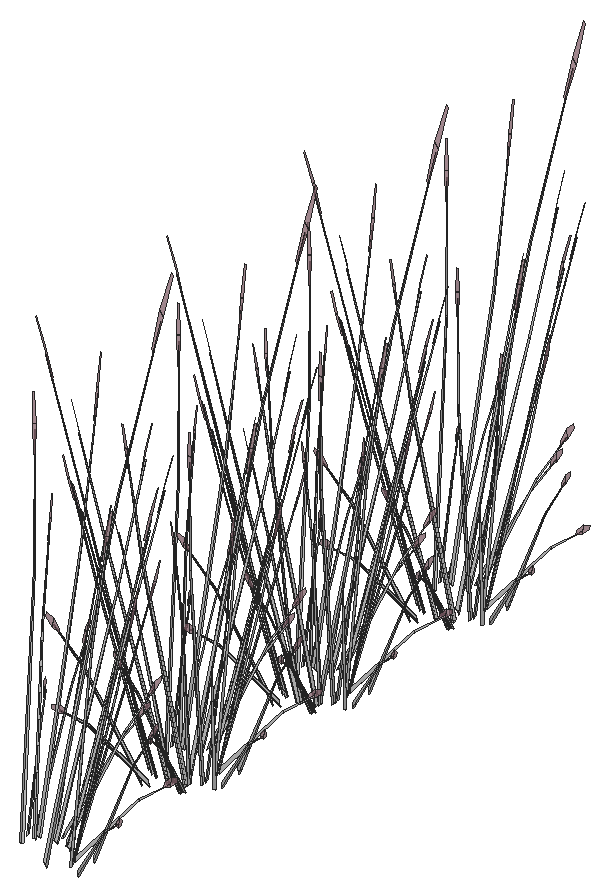
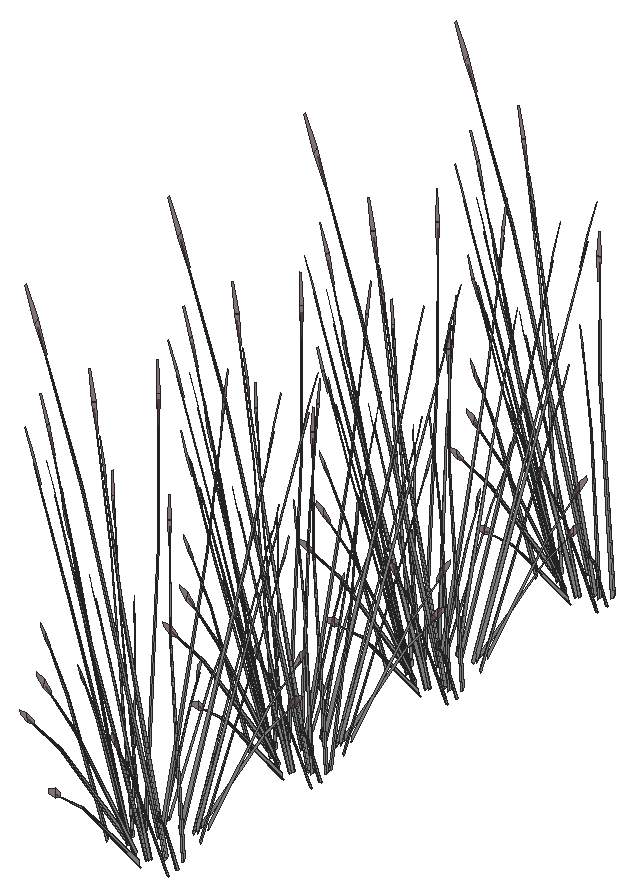
# SketchUp Ruby script. Lengths in inches.
U = 1.inch
M = Sketchup.active_model
def pt(a) = Geom::Point3d.new(a.map { |v| v * U })
def face(e, loops, mat)
  f = e.add_face(loops[0].map { |a| pt(a) })
  loops[1..].each { |l| e.add_face(l.map { |a| pt(a) }).erase! }
  f.material = f.back_material = mat if mat
  f
end
# faces: each face lists its corners as indices into pts; further lists are holes
def faces(e, pts, list, mat = nil) = list.each { |f| face(e, (f[0].is_a?(Array) ? f : [f]).map { |l| l.map { |i| pts[i] } }, mat) }
# xy, xz, yz: faces in a plane at the given z, y or x. An outline is a flat list of corners, or four numbers for a rectangle; further outlines are holes
def ring(l) = l.size == 4 ? [[l[0], l[1]], [l[2], l[1]], [l[2], l[3]], [l[0], l[3]]] : l.each_slice(2).to_a
def flat(e, list, mat, &to3) = list.each { |f| face(e, (f[0].is_a?(Array) ? f : [f]).map { |l| ring(l).map { |u, v| to3.(u, v) } }, mat) }
def xy(e, z, list, mat = nil) = flat(e, list, mat) { |x, y| [x, y, z] }
def xz(e, y, list, mat = nil) = flat(e, list, mat) { |x, z| [x, y, z] }
def yz(e, x, list, mat = nil) = flat(e, list, mat) { |y, z| [x, y, z] }
def lines(e, pts, list) = list.each { |a, b| e.add_line(pt(pts[a]), pt(pts[b])) }
# prism: a flat outline (further loops are holes) pulled along v
def prism(e, loops, v, mat = nil)
  f = face(e, loops, mat); d = Geom::Vector3d.new(v.map { |x| x * U })
  f.pushpull(f.normal.samedirection?(d) ? d.length : -d.length)
end
def box(e, o, s, mat = nil) = prism(e, [[o, [o[0] + s[0], o[1], o[2]], [o[0] + s[0], o[1] + s[1], o[2]], [o[0], o[1] + s[1], o[2]]]], [0, 0, s[2]], mat)
def at(x, y, z, deg = 0) = Geom::Transformation.translation(pt([x, y, z])) * Geom::Transformation.rotation(ORIGIN, Z_AXIS, deg.degrees)
def axes(o, x, y, z) = Geom::Transformation.new([*x, 0, *y, 0, *z, 0, *pt(o).to_a, 1])
def part(name) = M.definitions.add(name)
# library, detail: a bought-in or finely detailed component or shape, given as its bounding box
def library(name, o, s) = part(name).tap { |d| box(d.entities, o, s) }
def detail(e, o, s) = box(e.add_group.entities, o, s)
def put(e, d, t, mat = nil) = e.add_instance(d, t).tap { |i| i.material = mat if mat }
def group(e, t, mat = nil) = e.add_group.tap { |g| g.transformation = t; g.material = mat if mat }.entities
root = M.entities
M.materials.add("LightPink_Translucent").color = [144, 107, 117]
M.materials["LightPink_Translucent"].alpha = 0.75
M.materials.add("[_0053_Ivory_]").color = [200, 200, 200]
c1 = part("blade")
p = [[2.15,0.21,22],[0,0.17,0],[0.09,0.45,0],[2.18,0.31,22],[2.29,0.31,22],[0.38,0.45,0],
  [2.48,0.24,33],[2.49,0.24,33],[2.48,0.22,33]]
faces(c1.entities,p,[[0,1,2,3],[4,5,2,3],[6,3,4,7],[8,0,3,6]])
c2 = part("seeds")
p = [[0.3,-0.1,1.38],[-0.01,-0.03,1.59],[-0.01,-0.03,0.03],[0.14,-0.07,-0.07],[0.29,-0.03,3],[0.15,0.01,3.11]]
faces(c2.entities,p,[[0,1,2,3],[1,0,4,5]],"LightPink_Translucent")
c3 = part("blade with seeds")
put(c3.entities,c1,at(0,0,0))
put(c3.entities,c2,axes([2.4,0.25,30.99],[1.5799,-0.05474,1.17369],[-0.12525,1.92788,0.29478],[-0.07173,-0.02425,1.56792]))
put(root,c3,axes([648.13,153.46,131.37],[0.08428,-0.09579,1.74944],[-0.10787,-0.58756,-0.27667],[0.21147,-0.1114,0.14031]),"[_0053_Ivory_]")
put(root,c3,axes([646.47,154.35,131.6875],[-0.30559,-0.56943,-0.1216],[0.54237,-0.27983,-0.67495],[0.22856,-0.07513,1.02557]),"[_0053_Ivory_]")
put(root,c3,axes([646.72,154.34,131.38],[0.22307,0.42878,0.0643],[-0.40677,0.20987,0.50621],[0.17931,-0.04141,0.77189]),"[_0053_Ivory_]")
put(root,c3,axes([647.6875,156.04,131.36],[-0.05492,-0.05505,1.77383],[0.12013,-0.59013,-0.16761],[0.21632,-0.0377,0.31391]),"[_0053_Ivory_]")
put(root,c3,axes([645.79,155.53,131.6875],[0.03252,-0.63953,-0.1216],[0.61574,0.01748,-0.67495],[0.23714,0.04442,1.02557]),"[_0053_Ivory_]")
put(root,c3,axes([646.32,155.15,131.37],[0.13029,-0.01064,1.74944],[0.35737,-0.48855,-0.27667],[0.23175,0.06449,0.14031]),"[_0053_Ivory_]")
put(root,c3,axes([646.01,155.64,131.38],[-0.03058,0.47819,0.0643],[-0.4618,-0.01311,0.50621],[0.1769,0.05004,0.77189]),"[_0053_Ivory_]")
put(root,c3,axes([644.98,153.05,131.13],[-0.52482,-0.32674,1.38283],[0.55416,-0.50872,0.59665],[0.16933,0.30658,1.33663]),"[_0053_Ivory_]")
put(root,c3,axes([641.2,154.43,131.6875],[0.56181,0.34675,-0.1216],[-0.32367,0.50216,-0.67495],[-0.15873,0.17455,1.02557]),"[_0053_Ivory_]")
put(root,c3,axes([644.57,156.23,131.6875],[0.36191,-0.53827,-0.1216],[0.52412,0.3101,-0.67495],[0.18219,0.15207,1.02557]),"[_0053_Ivory_]")
put(root,c3,axes([644.1,156.68,131.36],[0.0018,-0.07613,1.77383],[0.52048,-0.3359,-0.16761],[0.18079,0.11989,0.31391]),"[_0053_Ivory_]")
put(root,c3,axes([641.82,155.8,131.38],[-0.49911,-0.0293,0.0643],[0.01368,-0.44245,0.50621],[-0.05223,0.16948,0.77189]),"[_0053_Ivory_]")
put(root,c3,axes([644.71,156.43,131.38],[-0.27604,0.39948,0.0643],[-0.39309,-0.23258,0.50621],[0.12709,0.12808,0.77189]),"[_0053_Ivory_]")
put(root,c3,axes([643.18,156.49,131.38],[-0.44753,0.21372,0.0643],[-0.21905,-0.38973,0.50621],[0.04322,0.1718,0.77189]),"[_0053_Ivory_]")
put(root,c3,axes([640.56,155.875,131.37],[-0.0151,0.12444,1.74944],[0.42844,0.43292,-0.27667],[-0.11216,0.20472,0.14031]),"[_0053_Ivory_]")
put(root,c3,axes([641.93,155.59,132.05],[0.6675,0.03116,-0.13498],[-0.01824,0.58993,-0.74919],[-0.04637,0.2272,1.13838]),"[_0053_Ivory_]")
put(root,c3,axes([643.16,156.25,131.6875],[0.59433,-0.29278,-0.1216],[0.29207,0.51964,-0.67495],[0.07842,0.21898,1.02557]),"[_0053_Ivory_]")
put(root,c3,axes([640.51,157.15,131.36],[0.0689,-0.03797,1.77383],[0.5695,0.25254,-0.16761],[-0.01338,0.21027,0.31391]),"[_0053_Ivory_]")
put(root,c3,axes([643.02,157.41,131.37],[0.07699,0.10127,1.74944],[0.6213,0.03978,-0.27667],[0.06248,0.22333,0.14031]),"[_0053_Ivory_]")
put(root,c3,axes([643.55,168.3,131.37],[-0.0929,-0.08817,1.74944],[-0.61994,0.0559,-0.27667],[-0.09894,-0.21089,0.14031]),"[_0053_Ivory_]")
put(root,c3,axes([646.33,169.38,131.37],[-0.00586,-0.12516,1.74944],[-0.49517,-0.36172,-0.27667],[0.07656,-0.21927,0.14031]),"[_0053_Ivory_]")
put(root,c3,axes([646.2,168.93,131.36],[-0.06168,0.04803,1.77383],[-0.60432,-0.16205,-0.16761],[-0.02188,-0.20961,0.31391]),"[_0053_Ivory_]")
put(root,c3,axes([642.91,168.01,131.36],[-0.01133,0.07538,1.77383],[-0.55883,0.27355,-0.16761],[-0.16445,-0.13983,0.31391]),"[_0053_Ivory_]")
put(root,c3,axes([644.49,169.66,131.6875],[-0.59433,0.29278,-0.1216],[-0.29207,-0.51964,-0.67495],[-0.07842,-0.21898,1.02557]),"[_0053_Ivory_]")
put(root,c3,axes([645.72,170.32,131.6875],[-0.6675,-0.03116,-0.1216],[0.01824,-0.58993,-0.67495],[0.04637,-0.2272,1.02557]),"[_0053_Ivory_]")
put(root,c3,axes([644.48,169.43,131.38],[0.44753,-0.21372,0.0643],[0.21905,0.38973,0.50621],[-0.04322,-0.1718,0.77189]),"[_0053_Ivory_]")
put(root,c3,axes([642.94,169.49,131.38],[0.27604,-0.39948,0.0643],[0.39309,0.23258,0.50621],[-0.12709,-0.12808,0.77189]),"[_0053_Ivory_]")
put(root,c3,axes([643.07,169.44,132.08],[-0.40534,0.60286,-0.13619],[-0.58702,-0.34732,-0.75594],[-0.20405,-0.17032,1.14864]),"[_0053_Ivory_]")
put(root,c3,axes([645.84,170.11,131.38],[0.49911,0.0293,0.0643],[-0.01368,0.44245,0.50621],[0.05223,-0.16948,0.77189]),"[_0053_Ivory_]")
put(root,c3,axes([646.45,171.48,131.6875],[-0.56181,-0.34675,-0.1216],[0.32367,-0.50216,-0.67495],[0.15873,-0.17455,1.02557]),"[_0053_Ivory_]")
put(root,c3,axes([647.83,171.33,131.36],[-0.07933,-0.00478,1.77383],[-0.32942,-0.51175,-0.16761],[0.13229,-0.16826,0.31391]),"[_0053_Ivory_]")
put(root,c3,axes([641.65,170.27,131.38],[0.03058,-0.47819,0.0643],[0.4618,0.01311,0.50621],[-0.1769,-0.05004,0.77189]),"[_0053_Ivory_]")
put(root,c3,axes([646.66,171.35,131.38],[0.41695,0.26447,0.0643],[-0.24275,0.37662,0.50621],[0.13368,-0.12176,0.77189]),"[_0053_Ivory_]")
put(root,c3,axes([648.13,171.94,131.37],[0.08428,-0.09579,1.74944],[-0.10787,-0.58756,-0.27667],[0.21147,-0.1114,0.14031]),"[_0053_Ivory_]")
put(root,c3,axes([646.47,172.83,131.6875],[-0.30559,-0.56943,-0.1216],[0.54237,-0.27983,-0.67495],[0.22856,-0.07513,1.02557]),"[_0053_Ivory_]")
put(root,c3,axes([646.72,172.82,131.38],[0.22307,0.42878,0.0643],[-0.40677,0.20987,0.50621],[0.17931,-0.04141,0.77189]),"[_0053_Ivory_]")
put(root,c3,axes([647.6875,174.53,131.36],[-0.05492,-0.05505,1.77383],[0.12013,-0.59013,-0.16761],[0.21632,-0.0377,0.31391]),"[_0053_Ivory_]")
put(root,c3,axes([645.79,174.02,131.6875],[0.03252,-0.63953,-0.1216],[0.61574,0.01748,-0.67495],[0.23714,0.04442,1.02557]),"[_0053_Ivory_]")
put(root,c3,axes([646.32,173.63,131.37],[0.13029,-0.01064,1.74944],[0.35737,-0.48855,-0.27667],[0.23175,0.06449,0.14031]),"[_0053_Ivory_]")
put(root,c3,axes([646.01,174.12,131.38],[-0.03058,0.47819,0.0643],[-0.4618,-0.01311,0.50621],[0.1769,0.05004,0.77189]),"[_0053_Ivory_]")
put(root,c3,axes([644.98,171.54,131.13],[-0.52482,-0.32674,1.38283],[0.55416,-0.50872,0.59665],[0.16933,0.30658,1.33663]),"[_0053_Ivory_]")
put(root,c3,axes([641.2,172.92,131.6875],[0.56181,0.34675,-0.1216],[-0.32367,0.50216,-0.67495],[-0.15873,0.17455,1.02557]),"[_0053_Ivory_]")
put(root,c3,axes([644.57,174.71,131.6875],[0.36191,-0.53827,-0.1216],[0.52412,0.3101,-0.67495],[0.18219,0.15207,1.02557]),"[_0053_Ivory_]")
put(root,c3,axes([644.1,175.16,131.36],[0.0018,-0.07613,1.77383],[0.52048,-0.3359,-0.16761],[0.18079,0.11989,0.31391]),"[_0053_Ivory_]")
put(root,c3,axes([641.82,174.29,131.38],[-0.49911,-0.0293,0.0643],[0.01368,-0.44245,0.50621],[-0.05223,0.16948,0.77189]),"[_0053_Ivory_]")
put(root,c3,axes([644.71,174.91,131.38],[-0.27604,0.39948,0.0643],[-0.39309,-0.23258,0.50621],[0.12709,0.12808,0.77189]),"[_0053_Ivory_]")
put(root,c3,axes([643.18,174.97,131.38],[-0.44753,0.21372,0.0643],[-0.21905,-0.38973,0.50621],[0.04322,0.1718,0.77189]),"[_0053_Ivory_]")
put(root,c3,axes([640.56,174.36,131.37],[-0.0151,0.12444,1.74944],[0.42844,0.43292,-0.27667],[-0.11216,0.20472,0.14031]),"[_0053_Ivory_]")
put(root,c3,axes([641.93,174.08,132.05],[0.6675,0.03116,-0.13498],[-0.01824,0.58993,-0.74919],[-0.04637,0.2272,1.13838]),"[_0053_Ivory_]")
put(root,c3,axes([643.16,174.73,131.6875],[0.59433,-0.29278,-0.1216],[0.29207,0.51964,-0.67495],[0.07842,0.21898,1.02557]),"[_0053_Ivory_]")
put(root,c3,axes([640.51,175.63,131.36],[0.0689,-0.03797,1.77383],[0.5695,0.25254,-0.16761],[-0.01338,0.21027,0.31391]),"[_0053_Ivory_]")
put(root,c3,axes([643.02,175.9,131.37],[0.07699,0.10127,1.74944],[0.6213,0.03978,-0.27667],[0.06248,0.22333,0.14031]),"[_0053_Ivory_]")
put(root,c3,axes([643.55,185.06,131.37],[-0.0929,-0.08817,1.74944],[-0.61994,0.0559,-0.27667],[-0.09894,-0.21089,0.14031]),"[_0053_Ivory_]")
put(root,c3,axes([646.33,186.14,131.37],[-0.00586,-0.12516,1.74944],[-0.49517,-0.36172,-0.27667],[0.07656,-0.21927,0.14031]),"[_0053_Ivory_]")
put(root,c3,axes([646.2,185.69,131.36],[-0.06168,0.04803,1.77383],[-0.60432,-0.16205,-0.16761],[-0.02188,-0.20961,0.31391]),"[_0053_Ivory_]")
put(root,c3,axes([642.91,184.77,131.36],[-0.01133,0.07538,1.77383],[-0.55883,0.27355,-0.16761],[-0.16445,-0.13983,0.31391]),"[_0053_Ivory_]")
put(root,c3,axes([644.49,186.42,131.6875],[-0.59433,0.29278,-0.1216],[-0.29207,-0.51964,-0.67495],[-0.07842,-0.21898,1.02557]),"[_0053_Ivory_]")
put(root,c3,axes([645.72,187.08,131.6875],[-0.6675,-0.03116,-0.1216],[0.01824,-0.58993,-0.67495],[0.04637,-0.2272,1.02557]),"[_0053_Ivory_]")
put(root,c3,axes([644.48,186.1875,131.38],[0.44753,-0.21372,0.0643],[0.21905,0.38973,0.50621],[-0.04322,-0.1718,0.77189]),"[_0053_Ivory_]")
put(root,c3,axes([642.94,186.25,131.38],[0.27604,-0.39948,0.0643],[0.39309,0.23258,0.50621],[-0.12709,-0.12808,0.77189]),"[_0053_Ivory_]")
put(root,c3,axes([643.07,186.2,132.08],[-0.40534,0.60286,-0.13619],[-0.58702,-0.34732,-0.75594],[-0.20405,-0.17032,1.14864]),"[_0053_Ivory_]")
put(root,c3,axes([645.84,186.87,131.38],[0.49911,0.0293,0.0643],[-0.01368,0.44245,0.50621],[0.05223,-0.16948,0.77189]),"[_0053_Ivory_]")
put(root,c3,axes([646.45,188.24,131.6875],[-0.56181,-0.34675,-0.1216],[0.32367,-0.50216,-0.67495],[0.15873,-0.17455,1.02557]),"[_0053_Ivory_]")
put(root,c3,axes([647.83,188.09,131.36],[-0.07933,-0.00478,1.77383],[-0.32942,-0.51175,-0.16761],[0.13229,-0.16826,0.31391]),"[_0053_Ivory_]")
put(root,c3,axes([641.65,187.03,131.38],[0.03058,-0.47819,0.0643],[0.4618,0.01311,0.50621],[-0.1769,-0.05004,0.77189]),"[_0053_Ivory_]")
put(root,c3,axes([646.66,188.11,131.38],[0.41695,0.26447,0.0643],[-0.24275,0.37662,0.50621],[0.13368,-0.12176,0.77189]),"[_0053_Ivory_]")
put(root,c3,axes([648.13,188.7,131.37],[0.08428,-0.09579,1.74944],[-0.10787,-0.58756,-0.27667],[0.21147,-0.1114,0.14031]),"[_0053_Ivory_]")
put(root,c3,axes([646.47,189.59,131.6875],[-0.30559,-0.56943,-0.1216],[0.54237,-0.27983,-0.67495],[0.22856,-0.07513,1.02557]),"[_0053_Ivory_]")
put(root,c3,axes([646.72,189.58,131.38],[0.22307,0.42878,0.0643],[-0.40677,0.20987,0.50621],[0.17931,-0.04141,0.77189]),"[_0053_Ivory_]")
put(root,c3,axes([647.6875,191.28,131.36],[-0.05492,-0.05505,1.77383],[0.12013,-0.59013,-0.16761],[0.21632,-0.0377,0.31391]),"[_0053_Ivory_]")
put(root,c3,axes([645.79,190.78,131.6875],[0.03252,-0.63953,-0.1216],[0.61574,0.01748,-0.67495],[0.23714,0.04442,1.02557]),"[_0053_Ivory_]")
put(root,c3,axes([646.32,190.39,131.37],[0.13029,-0.01064,1.74944],[0.35737,-0.48855,-0.27667],[0.23175,0.06449,0.14031]),"[_0053_Ivory_]")
put(root,c3,axes([641,189.8,131.38],[-0.41695,-0.26447,0.0643],[0.24275,-0.37662,0.50621],[-0.13368,0.12176,0.77189]),"[_0053_Ivory_]")
put(root,c3,axes([646.01,190.88,131.38],[-0.03058,0.47819,0.0643],[-0.4618,-0.01311,0.50621],[0.1769,0.05004,0.77189]),"[_0053_Ivory_]")
put(root,c3,axes([644.98,188.3,131.13],[-0.52482,-0.32674,1.38283],[0.55416,-0.50872,0.59665],[0.16933,0.30658,1.33663]),"[_0053_Ivory_]")
put(root,c3,axes([641.2,189.67,131.6875],[0.56181,0.34675,-0.1216],[-0.32367,0.50216,-0.67495],[-0.15873,0.17455,1.02557]),"[_0053_Ivory_]")
put(root,c3,axes([644.57,191.47,131.6875],[0.36191,-0.53827,-0.1216],[0.52412,0.3101,-0.67495],[0.18219,0.15207,1.02557]),"[_0053_Ivory_]")
put(root,c3,axes([644.1,191.92,131.36],[0.0018,-0.07613,1.77383],[0.52048,-0.3359,-0.16761],[0.18079,0.11989,0.31391]),"[_0053_Ivory_]")
put(root,c3,axes([641.82,191.05,131.38],[-0.49911,-0.0293,0.0643],[0.01368,-0.44245,0.50621],[-0.05223,0.16948,0.77189]),"[_0053_Ivory_]")
put(root,c3,axes([644.71,191.67,131.38],[-0.27604,0.39948,0.0643],[-0.39309,-0.23258,0.50621],[0.12709,0.12808,0.77189]),"[_0053_Ivory_]")
put(root,c3,axes([643.18,191.73,131.38],[-0.44753,0.21372,0.0643],[-0.21905,-0.38973,0.50621],[0.04322,0.1718,0.77189]),"[_0053_Ivory_]")
put(root,c3,axes([640.56,191.12,131.37],[-0.0151,0.12444,1.74944],[0.42844,0.43292,-0.27667],[-0.11216,0.20472,0.14031]),"[_0053_Ivory_]")
put(root,c3,axes([641.93,190.84,132.05],[0.6675,0.03116,-0.13498],[-0.01824,0.58993,-0.74919],[-0.04637,0.2272,1.13838]),"[_0053_Ivory_]")
put(root,c3,axes([643.16,191.49,131.6875],[0.59433,-0.29278,-0.1216],[0.29207,0.51964,-0.67495],[0.07842,0.21898,1.02557]),"[_0053_Ivory_]")
put(root,c3,axes([640.51,192.39,131.36],[0.0689,-0.03797,1.77383],[0.5695,0.25254,-0.16761],[-0.01338,0.21027,0.31391]),"[_0053_Ivory_]")
put(root,c3,axes([643.02,192.66,131.37],[0.07699,0.10127,1.74944],[0.6213,0.03978,-0.27667],[0.06248,0.22333,0.14031]),"[_0053_Ivory_]")
put(root,c3,axes([643.55,202.65,131.37],[-0.0929,-0.08817,1.74944],[-0.61994,0.0559,-0.27667],[-0.09894,-0.21089,0.14031]),"[_0053_Ivory_]")
put(root,c3,axes([646.33,203.73,131.37],[-0.00586,-0.12516,1.74944],[-0.49517,-0.36172,-0.27667],[0.07656,-0.21927,0.14031]),"[_0053_Ivory_]")
put(root,c3,axes([646.2,203.28,131.36],[-0.06168,0.04803,1.77383],[-0.60432,-0.16205,-0.16761],[-0.02188,-0.20961,0.31391]),"[_0053_Ivory_]")
put(root,c3,axes([642.91,202.36,131.36],[-0.01133,0.07538,1.77383],[-0.55883,0.27355,-0.16761],[-0.16445,-0.13983,0.31391]),"[_0053_Ivory_]")
put(root,c3,axes([644.49,204.01,131.6875],[-0.59433,0.29278,-0.1216],[-0.29207,-0.51964,-0.67495],[-0.07842,-0.21898,1.02557]),"[_0053_Ivory_]")
put(root,c3,axes([645.72,204.67,131.6875],[-0.6675,-0.03116,-0.1216],[0.01824,-0.58993,-0.67495],[0.04637,-0.2272,1.02557]),"[_0053_Ivory_]")
put(root,c3,axes([642.94,203.84,131.38],[0.27604,-0.39948,0.0643],[0.39309,0.23258,0.50621],[-0.12709,-0.12808,0.77189]),"[_0053_Ivory_]")
put(root,c3,axes([643.07,203.8,132.08],[-0.40534,0.60286,-0.13619],[-0.58702,-0.34732,-0.75594],[-0.20405,-0.17032,1.14864]),"[_0053_Ivory_]")
put(root,c3,axes([646.45,205.83,131.6875],[-0.56181,-0.34675,-0.1216],[0.32367,-0.50216,-0.67495],[0.15873,-0.17455,1.02557]),"[_0053_Ivory_]")
put(root,c3,axes([647.83,205.68,131.36],[-0.07933,-0.00478,1.77383],[-0.32942,-0.51175,-0.16761],[0.13229,-0.16826,0.31391]),"[_0053_Ivory_]")
put(root,c3,axes([641.65,204.625,131.38],[0.03058,-0.47819,0.0643],[0.4618,0.01311,0.50621],[-0.1769,-0.05004,0.77189]),"[_0053_Ivory_]")
put(root,c3,axes([646.66,205.7,131.38],[0.41695,0.26447,0.0643],[-0.24275,0.37662,0.50621],[0.13368,-0.12176,0.77189]),"[_0053_Ivory_]")
put(root,c3,axes([648.13,206.29,131.37],[0.08428,-0.09579,1.74944],[-0.10787,-0.58756,-0.27667],[0.21147,-0.1114,0.14031]),"[_0053_Ivory_]")
put(root,c3,axes([646.47,207.18,131.6875],[-0.30559,-0.56943,-0.1216],[0.54237,-0.27983,-0.67495],[0.22856,-0.07513,1.02557]),"[_0053_Ivory_]")
put(root,c3,axes([646.72,207.17,131.38],[0.22307,0.42878,0.0643],[-0.40677,0.20987,0.50621],[0.17931,-0.04141,0.77189]),"[_0053_Ivory_]")
put(root,c3,axes([647.6875,208.875,131.36],[-0.05492,-0.05505,1.77383],[0.12013,-0.59013,-0.16761],[0.21632,-0.0377,0.31391]),"[_0053_Ivory_]")
put(root,c3,axes([645.79,208.37,131.6875],[0.03252,-0.63953,-0.1216],[0.61574,0.01748,-0.67495],[0.23714,0.04442,1.02557]),"[_0053_Ivory_]")
put(root,c3,axes([646.32,207.98,131.37],[0.13029,-0.01064,1.74944],[0.35737,-0.48855,-0.27667],[0.23175,0.06449,0.14031]),"[_0053_Ivory_]")
put(root,c3,axes([644.98,205.89,131.13],[-0.52482,-0.32674,1.38283],[0.55416,-0.50872,0.59665],[0.16933,0.30658,1.33663]),"[_0053_Ivory_]")
put(root,c3,axes([641.2,207.27,131.6875],[0.56181,0.34675,-0.1216],[-0.32367,0.50216,-0.67495],[-0.15873,0.17455,1.02557]),"[_0053_Ivory_]")
put(root,c3,axes([644.57,209.0625,131.6875],[0.36191,-0.53827,-0.1216],[0.52412,0.3101,-0.67495],[0.18219,0.15207,1.02557]),"[_0053_Ivory_]")
put(root,c3,axes([644.1,209.51,131.36],[0.0018,-0.07613,1.77383],[0.52048,-0.3359,-0.16761],[0.18079,0.11989,0.31391]),"[_0053_Ivory_]")
put(root,c3,axes([643.18,209.32,131.38],[-0.44753,0.21372,0.0643],[-0.21905,-0.38973,0.50621],[0.04322,0.1718,0.77189]),"[_0053_Ivory_]")
put(root,c3,axes([640.56,208.71,131.37],[-0.0151,0.12444,1.74944],[0.42844,0.43292,-0.27667],[-0.11216,0.20472,0.14031]),"[_0053_Ivory_]")
put(root,c3,axes([641.93,208.43,132.05],[0.6675,0.03116,-0.13498],[-0.01824,0.58993,-0.74919],[-0.04637,0.2272,1.13838]),"[_0053_Ivory_]")
put(root,c3,axes([643.16,209.08,131.6875],[0.59433,-0.29278,-0.1216],[0.29207,0.51964,-0.67495],[0.07842,0.21898,1.02557]),"[_0053_Ivory_]")
put(root,c3,axes([640.51,209.98,131.36],[0.0689,-0.03797,1.77383],[0.5695,0.25254,-0.16761],[-0.01338,0.21027,0.31391]),"[_0053_Ivory_]")
put(root,c3,axes([643.02,210.25,131.37],[0.07699,0.10127,1.74944],[0.6213,0.03978,-0.27667],[0.06248,0.22333,0.14031]),"[_0053_Ivory_]")
